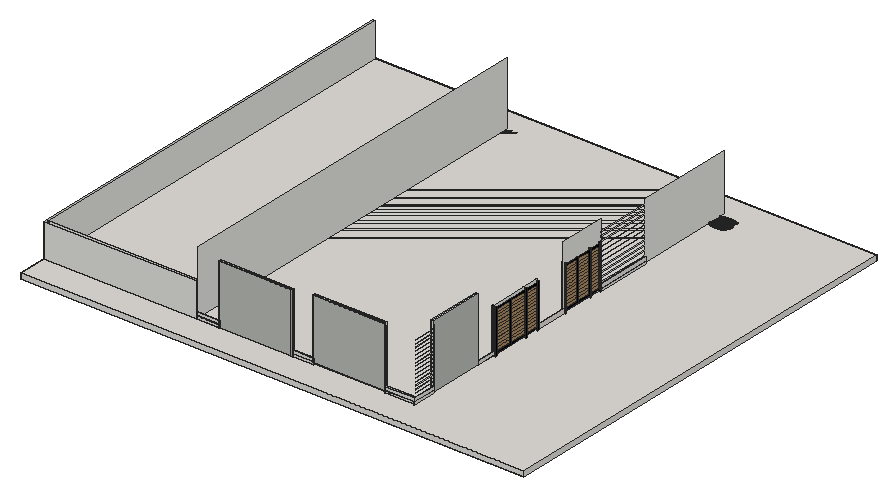
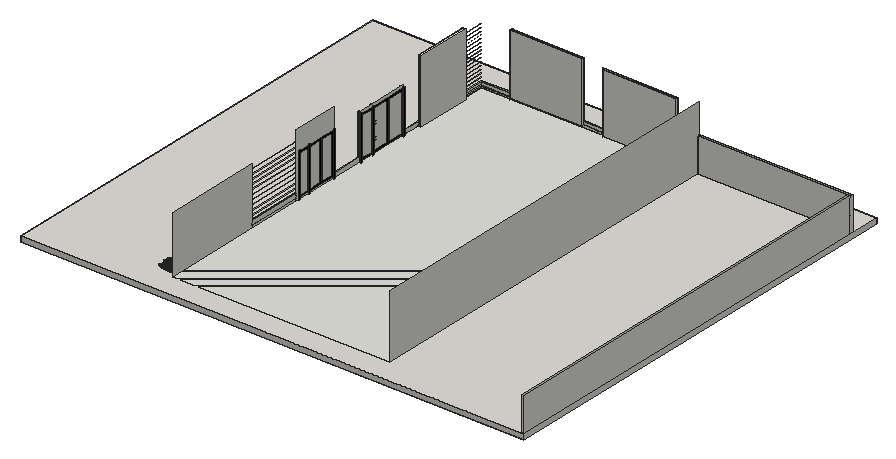
# SketchUp Ruby script. Lengths in inches.
U = 1.inch
M = Sketchup.active_model
def pt(a) = Geom::Point3d.new(a.map { |v| v * U })
def face(e, loops, mat)
  f = e.add_face(loops[0].map { |a| pt(a) })
  loops[1..].each { |l| e.add_face(l.map { |a| pt(a) }).erase! }
  f.material = f.back_material = mat if mat
  f
end
# faces: each face lists its corners as indices into pts; further lists are holes
def faces(e, pts, list, mat = nil) = list.each { |f| face(e, (f[0].is_a?(Array) ? f : [f]).map { |l| l.map { |i| pts[i] } }, mat) }
# xy, xz, yz: faces in a plane at the given z, y or x. An outline is a flat list of corners, or four numbers for a rectangle; further outlines are holes
def ring(l) = l.size == 4 ? [[l[0], l[1]], [l[2], l[1]], [l[2], l[3]], [l[0], l[3]]] : l.each_slice(2).to_a
def flat(e, list, mat, &to3) = list.each { |f| face(e, (f[0].is_a?(Array) ? f : [f]).map { |l| ring(l).map { |u, v| to3.(u, v) } }, mat) }
def xy(e, z, list, mat = nil) = flat(e, list, mat) { |x, y| [x, y, z] }
def xz(e, y, list, mat = nil) = flat(e, list, mat) { |x, z| [x, y, z] }
def yz(e, x, list, mat = nil) = flat(e, list, mat) { |y, z| [x, y, z] }
def lines(e, pts, list) = list.each { |a, b| e.add_line(pt(pts[a]), pt(pts[b])) }
# prism: a flat outline (further loops are holes) pulled along v
def prism(e, loops, v, mat = nil)
  f = face(e, loops, mat); d = Geom::Vector3d.new(v.map { |x| x * U })
  f.pushpull(f.normal.samedirection?(d) ? d.length : -d.length)
end
def box(e, o, s, mat = nil) = prism(e, [[o, [o[0] + s[0], o[1], o[2]], [o[0] + s[0], o[1] + s[1], o[2]], [o[0], o[1] + s[1], o[2]]]], [0, 0, s[2]], mat)
def at(x, y, z, deg = 0) = Geom::Transformation.translation(pt([x, y, z])) * Geom::Transformation.rotation(ORIGIN, Z_AXIS, deg.degrees)
def axes(o, x, y, z) = Geom::Transformation.new([*x, 0, *y, 0, *z, 0, *pt(o).to_a, 1])
def part(name) = M.definitions.add(name)
# library, detail: a bought-in or finely detailed component or shape, given as its bounding box
def library(name, o, s) = part(name).tap { |d| box(d.entities, o, s) }
def detail(e, o, s) = box(e.add_group.entities, o, s)
def put(e, d, t, mat = nil) = e.add_instance(d, t).tap { |i| i.material = mat if mat }
def group(e, t, mat = nil) = e.add_group.tap { |g| g.transformation = t; g.material = mat if mat }.entities
root = M.entities
M.materials.add("CarPaint_Matte_Black").color = [3, 3, 3]
M.materials.add("MaquetteWood_B01_12cm").color = [171, 138, 99]
M.materials.add("Material10").color = [48, 100, 38]
M.materials.add("Material3").color = [68, 110, 58]
M.materials.add("Material4").color = [48, 90, 38]
M.materials.add("Material5").color = [68, 110, 48]
M.materials.add("Material6").color = [48, 90, 48]
M.materials.add("Material7").color = [58, 110, 58]
M.materials.add("Material8").color = [58, 90, 38]
M.materials.add("Material9").color = [68, 100, 58]
M.materials.add("PJ_WallGraphic_V2").color = [185, 188, 181]
M.materials.add("[Terrazzo Tile Accent]").color = [224, 221, 217]
c1 = part("Component\#17")
prism(c1.entities,[[[51.57,0,-2.36],[0,0.39,-2.36],[0.07,5.78,-2.36],[51.65,5.38,-2.36]]],[0,0,82.68])
c2 = part("Component\#14")
prism(c2.entities,[[[1.98,0.39,-2.36],[37.4,0.02,-2.36],[37.4,-0.1,-2.36],[1.98,0.28,-2.36]]],[0,0,82.68],"PJ_WallGraphic_V2")
put(c2.entities,c1,axes([1.98,0,0],[0.68667,0,0],[0,1,0],[0,0,1]))
c3 = part("Gate post")
prism(c3.entities,[[[0,0,0],[3.9375,0,0],[3.9375,0,3.9375],[3.9375,0,98.43],[0,0,98.43]]],[0,7.875,0],"CarPaint_Matte_Black")
c4 = part("Gate post \#2")
box(c4.entities,[0,0,0],[3.9375,7.875,98.43],"CarPaint_Matte_Black")
c5 = part("Gate post \#1")
prism(c5.entities,[[[0,0,0],[3.9375,0,0],[3.9375,0,3.9375],[3.9375,0,98.43],[0,0,98.43]]],[0,7.875,0],"CarPaint_Matte_Black")
c6 = part("Gate leaf frame \#1")
prism(c6.entities,[[[57.09,3.9375,3.9375],[1.97,3.9375,3.9375],[1.97,3.9375,94.49],[57.09,3.9375,94.49]],[[54.13,3.9375,6.89],[54.13,3.9375,91.54],[4.92,3.9375,91.54],[4.92,3.9375,6.89]]],[0,-3.86,0],"CarPaint_Matte_Black")
c7 = part("Gate slat \#1")
box(c7.entities,[0,0,0],[49.21,1.18,5.91],"MaquetteWood_B01_12cm")
c8 = part("Slatted gate panel")
put(c8.entities,c7,at(0,0,25.2))
put(c8.entities,c7,at(0,0,44.09))
put(c8.entities,c7,at(0,0,75.59))
put(c8.entities,c7,at(0,0,69.29))
put(c8.entities,c7,at(0,0,18.9))
put(c8.entities,c7,at(0,0,56.69))
put(c8.entities,c7,at(0,0,50.39))
put(c8.entities,c7,at(0,0,12.6))
put(c8.entities,c7,at(0,0,6.3))
put(c8.entities,c7,at(0,0,37.8))
put(c8.entities,c7,at(0,0,0))
put(c8.entities,c7,at(0,0,31.5))
put(c8.entities,c7,at(0,0,62.99))
c9 = part("Gate leaf frame")
prism(c9.entities,[[[0.98,0,3.9375],[76.39,0,3.9375],[76.39,0,94.49],[0.98,0,94.49]],[[73.43,0,6.89],[3.9375,0,6.89],[3.9375,0,91.54],[73.43,0,91.54]]],[0,3.86,0],"CarPaint_Matte_Black")
c10 = part("Gate slat")
box(c10.entities,[0,0,0],[69.5,1.18,5.91],"MaquetteWood_B01_12cm")
c11 = part("Gate infill panel")
put(c11.entities,c10,at(0,0,56.69))
put(c11.entities,c10,at(0,0,12.6))
put(c11.entities,c10,at(0,0,18.9))
put(c11.entities,c10,at(0,0,37.8))
put(c11.entities,c10,at(0,0,6.3))
put(c11.entities,c10,at(0,0,25.2))
put(c11.entities,c10,at(0,0,75.59))
put(c11.entities,c10,at(0,0,44.09))
put(c11.entities,c10,at(0,0,50.39))
put(c11.entities,c10,at(0,0,0))
put(c11.entities,c10,at(0,0,31.5))
put(c11.entities,c10,at(0,0,62.99))
put(c11.entities,c10,at(0,0,69.29))
c12 = part("Entrance gate assembly")
put(c12.entities,c3,at(0,0,0))
put(c12.entities,c4,at(223.64,0,0))
put(c12.entities,c5,at(160.64,0,0))
g1 = group(c12.entities,at(166.55,2.04,3.9375))
put(g1,c6,at(-1.97,-0.07,-3.9375))
put(g1,c8,at(2.95,1.34,4.33))
g2 = group(c12.entities,at(83.27,2.04,3.9375))
put(g2,c9,at(-0.98,0,-3.9375))
put(g2,c11,at(2.95,1.34,4.33))
g3 = group(c12.entities,at(5.91,2.04,3.9375))
put(g3,c9,axes([76.39,0,-3.9375],[-1,0,0],[0,1,0],[0,0,1]))
put(g3,c11,axes([72.45,1.34,4.33],[-1,0,0],[0,1,0],[0,0,1]))
c13 = part("grass00")
p = [[-0.6875,0.15,0],[-0.56,0.08,5.52],[-0.04,0.03,2.76],[0.48,-0.02,0],[0.35,-0.02,5.52],[-0.1,-0.14,5.52],
  [-0.12,0.65,8.37],[-0.42,0.65,8.37]]
faces(c13.entities,p,[[0,1,2,3],[3,2,4],[1,5,2],[5,4,2],[1,6,5],[4,5,6],[7,6,1]])
c14 = part("Group16\#1")
put(c14.entities,c13,axes([1.44,-0.61,-0.01],[0.05352,0.12609,0],[-0.10704,0.04543,0.07239],[0.06664,-0.02828,0.11628]),"Material6")
put(c14.entities,c13,axes([0.76,-0.15,-0.01],[0.04676,0.24062,0],[-0.23162,0.04501,0.06642],[0.0652,-0.01267,0.23595]),"Material3")
put(c14.entities,c13,axes([0.79,0.01,-0.01],[-0.00606,0.34651,0],[-0.34381,-0.00602,0.0432],[0.04319,0.00076,0.34386]))
put(c14.entities,c13,axes([1,0.23,-0.01],[-0.07192,0.31144,0],[-0.28722,-0.06632,0.1236],[0.12043,0.02781,0.29478]),"Material5")
put(c14.entities,c13,axes([1.66,0.77,-0.01],[-0.13828,0.29651,0],[-0.21551,-0.1005,0.22471],[0.20365,0.09498,0.23779]),"Material10")
put(c14.entities,c13,axes([0.6875,0.52,-0.01],[-0.18126,0.24051,0],[-0.22746,-0.17142,0.09788],[0.07817,0.05891,0.28481]),"Material5")
put(c14.entities,c13,axes([0.68,0.78,-0.01],[-0.215,0.18688,0],[-0.12385,-0.14248,0.21334],[0.13995,0.16101,0.18878]),"Material3")
put(c14.entities,c13,axes([0.56,1,-0.01],[-0.13756,0.07624,0],[-0.06159,-0.11112,0.0927],[0.04494,0.08108,0.12705]),"Material5")
put(c14.entities,c13,axes([0.2,0.64,-0.01],[-0.23729,0.07254,0],[-0.05711,-0.18681,0.153],[0.04473,0.14632,0.19535]),"Material10")
put(c14.entities,c13,axes([0.0625,0.72,-0.01],[-0.28874,0.02525,0],[-0.02179,-0.24916,0.14647],[0.01276,0.14591,0.25012]),"Material3")
put(c14.entities,c13,axes([-0.08,0.62,-0.01],[-0.34089,-0.04187,0],[0.03255,-0.26504,0.216],[-0.02633,0.21439,0.26703]),"Material10")
put(c14.entities,c13,axes([-0.34,0.98,-0.01],[-0.14314,-0.0493,0],[0.04397,-0.12769,0.06843],[-0.02228,0.0647,0.13505]),"Material10")
put(c14.entities,c13,axes([-0.87,1.45,-0.01],[-0.23488,-0.14114,0],[0.13761,-0.22901,0.06087],[-0.03135,0.05217,0.26717]))
put(c14.entities,c13,axes([-0.72,0.77,-0.01],[-0.14208,-0.13251,0],[0.07209,-0.0773,0.16301],[-0.11118,0.11922,0.1057]),"Material10")
put(c14.entities,c13,axes([-0.62,0.43,-0.01],[-0.14845,-0.21203,0],[0.18654,-0.13061,0.12304],[-0.10079,0.07057,0.22772]),"Material3")
put(c14.entities,c13,axes([-0.68,0.29,-0.01],[-0.13639,-0.32136,0],[0.31723,-0.13464,0.05579],[-0.05136,0.0218,0.34462]),"Material4")
put(c14.entities,c13,axes([-0.64,0.125,-0.01],[-0.0458,-0.23569,0],[0.22124,-0.043,0.08276],[-0.08124,0.01579,0.22538]),"Material7")
put(c14.entities,c13,axes([-1.6,-0.03,-0.01],[0.00576,-0.32897,0],[0.27526,0.00482,0.18018],[-0.18015,-0.00315,0.2753]),"Material5")
put(c14.entities,c13,axes([-1.36,-0.31,-0.01],[0.05718,-0.24765,0],[0.18172,0.04196,0.17267],[-0.16825,-0.03885,0.1865]),"Material10")
put(c14.entities,c13,axes([-1.54,-0.72,-0.01],[0.06537,-0.14017,0],[0.13555,0.06321,0.03939],[-0.0357,-0.01665,0.14956]))
put(c14.entities,c13,axes([-1.19,-0.9,-0.01],[0.09597,-0.12735,0],[0.11214,0.08451,0.07557],[-0.06035,-0.04548,0.14042]),"Material9")
put(c14.entities,c13,axes([-0.47,-0.54,-0.01],[0.11588,-0.10072,0],[0.0618,0.0711,0.12124],[-0.07953,-0.0915,0.0942]))
put(c14.entities,c13,axes([-0.47,-0.84,-0.01],[0.11927,-0.0661,0],[0.06603,0.11913,0.00646],[-0.00313,-0.00565,0.13621]),"Material5")
put(c14.entities,c13,axes([-0.38,-1.24,-0.01],[0.28037,-0.08571,0],[0.0618,0.20215,0.20315],[-0.05939,-0.19428,0.21139]),"Material9")
put(c14.entities,c13,axes([-0.06,-0.66,-0.01],[0.22719,-0.01987,0],[0.01247,0.14255,0.17758],[-0.01547,-0.17691,0.1431]),"Material8")
put(c14.entities,c13,axes([0.11,-0.89,-0.01],[0.14882,0.01828,0],[-0.01058,0.08611,0.12229],[0.01491,-0.12138,0.08676]),"Material6")
put(c14.entities,c13,axes([0.25,-0.72,-0.01],[0.20481,0.07053,0],[-0.06206,0.18022,0.10291],[0.03351,-0.0973,0.1906]),"Material6")
put(c14.entities,c13,axes([0.85,-1.42,-0.01],[0.16481,0.09904,0],[-0.09472,0.15762,0.05616],[0.02893,-0.04814,0.18389]),"Material5")
put(c14.entities,c13,axes([1.01,-1.09,-0.01],[0.21858,0.20385,0],[-0.17495,0.1876,0.15339],[0.10462,-0.11218,0.25652]),"Material10")
put(c14.entities,c13,axes([1.01,-0.71,-0.01],[0.08733,0.12473,0],[-0.06445,0.04512,0.13037],[0.1068,-0.07477,0.07867]),"Material6")
c15 = part("Group15\#1")
put(c15.entities,c14,at(0,0,0))
c16 = part("3darcstudiotree_grass00\#1")
put(c16.entities,c15,at(0,0,0))
xy(root,-5.37,[[814.625,599,817.6875,719.91]])
xy(root,-3.47,[[750.91,87.66,750.91,90.47,814.625,90.47,814.625,140.66,816.1875,140.66,816.1875,87.66]])
xy(root,-1.41,[[547.16,87.66,593.34,90.47]])
xy(root,-0.49,[[814.625,423.33,816.875,495.84]])
xy(root,0,[[336.5625,90.47,814.625,939.04]])
xy(root,0.07,[[336.5625,87.66,386.78,90.47]])
xy(root,0.9375,[[814.625,263.05,816.1875,305.04]])
xy(root,3.71,[[750.91,87.66,816.1875,87.66,816.1875,140.66,814.625,140.66,814.625,90.47,750.91,90.47]])
xy(root,3.79,[[814.625,599,817.6875,719.91]])
xy(root,4.59,[[750.91,87.66,750.91,90.47,814.625,90.47,814.625,140.66,816.1875,140.66,816.1875,87.66]])
xy(root,4.76,[[814.625,599,817.6875,719.91]])
xy(root,5.07,[[547.16,87.66,593.34,90.47]])
xy(root,5.21,[[547.16,87.66,593.34,90.47]])
xy(root,6.29,[[336.5625,87.66,386.78,90.47]])
xy(root,6.63,[[336.5625,87.66,386.78,90.47]])
xz(root,87.66,[[0.875,-0.51,0.75,73.42,336.43,74,336.5625,0.07]])
xz(root,87.66,[[750.91,-3.47,816.1875,3.71],[547.16,-1.41,593.34,5.07],[336.5625,0.07,386.78,6.29],[750.91,4.59,816.1875,11.77],[547.16,5.21,593.34,11.69],
  [336.5625,6.63,386.78,12.86]],"[Terrazzo Tile Accent]")
xz(root,90.47,[[336.5625,0,386.78,0.07],[386.78,0,547.16,131.62],[547.16,0,593.34,5.07],[593.34,0,750.91,131.62],[750.91,0,814.625,3.71],
  [336.5625,0.07,386.78,6.29],[750.91,3.71,814.625,4.59],[750.91,4.59,814.625,11.77],[547.16,5.07,593.34,5.21],[547.16,5.21,593.34,11.69],
  [336.5625,6.29,386.78,6.63],[336.5625,6.63,386.78,12.86]])
xz(root,94.42,[[0.875,-0.51,6.22,-0.5,6.1,73.43,0.75,73.42],[6.22,-0.5,336.5625,0.07,336.43,74,6.1,73.43]])
xz(root,140.66,[[814.625,-3.47,816.1875,0],[814.625,0,816.1875,3.71],[814.625,4.59,816.1875,11.77]])
xz(root,263.05,[[814.625,0.9375,816.1875,8.42]])
xz(root,305.04,[[814.625,0.9375,816.1875,8.42]])
xz(root,423.33,[[814.625,-0.49,816.875,8.5]])
xz(root,599,[[814.625,-5.37,817.6875,3.79],[814.625,4.76,817.6875,13.92]])
xz(root,719.91,[[814.625,-5.37,817.6875,3.79],[814.625,4.76,817.6875,13.92]])
yz(root,336.5625,[[90.47,0,939.04,140.0625],[87.66,0.07,90.47,6.29],[87.66,6.63,90.47,12.86]])
yz(root,386.78,[[87.66,0.07,90.47,6.29],[87.66,6.63,90.47,12.86]])
yz(root,547.16,[[87.66,-1.41,90.47,5.07],[87.66,5.21,90.47,11.69]])
yz(root,593.34,[[87.66,-1.41,90.47,5.07],[87.66,5.21,90.47,11.69]])
yz(root,750.91,[[87.66,-3.47,90.47,3.71],[87.66,4.59,90.47,11.77]])
yz(root,814.625,[[87.66,-3.47,87.66,3.71,90.47,3.71,90.47,0,140.66,0,140.66,-3.47],[140.66,0,140.91,0,140.91,131.62,140.66,131.62,140.66,125.4,90.47,125.4,90.47,125.11,140.66,125.11,140.66,117.93,90.47,117.93,90.47,117.55,140.66,117.55,140.66,110.36,90.47,110.36,90.47,110.05,140.66,110.05,140.66,102.86,90.47,102.86,90.47,102.61,140.66,102.61,140.66,95.43,90.47,95.43,90.47,95.17,140.66,95.17,140.66,87.99,90.47,87.99,90.47,87.67,140.66,87.67,140.66,80.49,90.47,80.49,90.47,80.21,140.66,80.21,140.66,73.03,90.47,73.03,90.47,72.77,140.66,72.77,140.66,65.59,90.47,65.59,90.47,65.33,140.66,65.33,140.66,58.15,90.47,58.15,90.47,57.77,140.66,57.77,140.66,50.59,90.47,50.59,90.47,50.15,140.66,50.15,140.66,42.96,90.47,42.96,90.47,42.52,140.66,42.52,140.66,35.34,90.47,35.34,90.47,34.9,140.66,34.9,140.66,27.71,90.47,27.71,90.47,27.27,140.66,27.27,140.66,20.09,90.47,20.09,90.47,19.58,140.66,19.58,140.66,12.4,90.47,12.4,90.47,11.77,140.66,11.77,140.66,4.59,90.47,4.59,90.47,3.71,140.66,3.71],[90.47,0,140.66,3.71],[140.91,0,263.05,131.62],[263.05,0,305.04,0.29],
  [305.04,0,423.33,98.4375],[423.33,0,495.84,8.5],[495.84,0,599,140.0625],[599,0,719.91,3.79],[719.91,0,939.04,0,939.04,125.29,719.91,125.29,719.91,116.13,599,116.13,599,115.17,719.91,115.17,719.91,106.01,599,106.01,599,105.04,719.91,105.04,719.91,95.88,599,95.88,599,94.92,719.91,94.92,719.91,85.76,599,85.76,599,84.79,719.91,84.79,719.91,75.63,599,75.63,599,74.67,719.91,74.67,719.91,65.51,599,65.51,599,64.54,719.91,64.54,719.91,55.38,599,55.38,599,54.42,719.91,54.42,719.91,45.26,599,45.26,599,44.29,719.91,44.29,719.91,35.13,599,35.13,599,34.17,719.91,34.17,719.91,25.01,599,25.01,599,24.04,719.91,24.04,719.91,14.88,599,14.88,599,13.92,719.91,13.92,719.91,4.76,599,4.76,599,3.79,719.91,3.79],
  [263.05,0.29,305.04,0.9375],[263.05,0.9375,305.04,8.42],[90.47,4.59,140.66,11.77],[599,4.76,719.91,13.92]])
yz(root,816.1875,[[87.66,-3.47,140.66,3.71],[263.05,0.9375,305.04,8.42],[87.66,4.59,140.66,11.77]],"[Terrazzo Tile Accent]")
yz(root,816.875,[[423.33,-0.49,495.84,8.5]],"[Terrazzo Tile Accent]")
yz(root,817.6875,[[599,-5.37,719.91,3.79],[599,4.76,719.91,13.92]],"[Terrazzo Tile Accent]")
p = [[0.875,87.66,-0.51],[0.875,94.42,-0.51],[0.75,94.42,73.42],[0.75,87.66,73.42],[0.75,990.97,73.42],[0.875,990.97,-0.51],
  [6.22,94.42,-0.5],[6.22,990.97,-0.5],[6.1,94.42,73.43],[6.1,990.97,73.43],[336.5625,90.47,0.07],[336.5625,87.66,0.07],
  [336.43,87.66,74],[336.43,90.47,74],[336.5625,94.42,0.07],[336.43,94.42,74],[814.625,305.04,0.29],[816.1875,305.04,0.29],
  [814.625,263.05,0.29],[816.1875,263.05,0.29],[6.1,94.42,0]]
faces(root,p,[[0,1,2,3],[1,2,4,5],[6,1,5,7],[8,6,7,9],[10,11,12,13],[14,10,13,15]])
lines(root,p,[[16,17],[18,19],[20,8]])
put(root,c2,axes([376.16,87.76,1.42],[4.494,0,0],[0,1,0],[0,0,1.60205]))
g4 = group(root,at(336.5625,690.47,-12),"[Terrazzo Tile Accent]")
box(g4,[-336.5625,-667.1875,0],[1107.6875,967.6875,12])
put(root,c2,axes([582.64,87.76,7.49],[4.494,0,0],[0,1,0],[0,0,1.60205]))
put(root,c2,axes([814.9,133.37,4],[0,3.46347,0],[-1,0,0],[0,0,1.69406]))
put(root,c12,axes([819.375,305.93,-1.54],[0,0.52,0],[-1,0,0],[0,0,1]))
put(root,c12,axes([819.48,497.55,0],[0,0.4264,0],[-1,0,0],[0,0,1]))
put(root,c16,axes([830.35,906.53,0],[-1.46443,-0.98467,0],[4.53365,-0.42141,-0.02925],[0.15457,-0.01437,1.7044]))
put(root,c16,axes([830.39,898.64,0],[-4.82729,-0.45997,0],[1.31646,-0.86349,-0.04688],[0.11487,-0.07535,1.58936]))
put(root,c16,axes([830.52,899.77,0],[-5.02983,-0.31612,0],[0.92163,-0.91652,-0.02201],[0.03056,-0.03039,1.34565]))
put(root,c16,axes([830.81,923.875,0],[-1.60248,-1.17219,0],[4.18284,-0.35739,-0.03013],[0.15857,-0.01355,1.53631]))
put(root,c16,axes([829.42,893.97,0],[4,0,0],[0,1,0],[0,0,1]))
put(root,c16,axes([829.67,923.15,0],[3.56901,0.48429,0],[-2.2351,1.02948,-0.01651],[-0.0487,0.02243,1.81134]))
put(root,c16,axes([830.52,907.96,0],[-2.03185,0.95693,0],[-3.64296,-0.48344,-0.02935],[-0.13306,-0.01766,1.32321]))
put(root,c16,axes([830.57,901.96,0],[3.55456,-0.14349,0],[0.62802,0.97236,-0.03713],[0.03348,0.05184,1.39317]))
put(root,c16,axes([830.98,921.17,0],[3.6372,-0.13455,0],[0.71258,1.2039,-0.00326],[0.00297,0.00501,1.88794]))
put(root,c16,axes([830.86,895.43,0],[1.65013,1.13441,0],[-3.55007,0.32275,-0.03897],[-0.23777,0.02162,1.53286]))
put(root,c16,axes([833.14,925.85,0],[-5.16631,0.09452,0],[-0.34124,-1.1657,-0.0067],[-0.00219,-0.00748,1.30916]))
put(root,c16,axes([833.88,895.84,0],[2.49255,-0.69469,0],[3.67207,0.82346,-0.03873],[0.17763,0.03983,1.89965]))
put(root,c16,axes([834.4,916.57,0],[-3.93651,0.31096,0],[-1.27927,-1.01217,-0.02199],[-0.03758,-0.02973,1.50537]))
put(root,c16,axes([834.38,913.66,0],[2.99864,-0.87357,0],[3.91675,0.8403,-0.00643],[0.02559,0.00549,1.6911]))
put(root,c16,axes([833.68,906.43,0],[0.74164,0.96677,0],[-4.8523,0.23265,-0.00068],[-0.00352,0.00017,1.62852]))
put(root,c16,axes([835.27,919.3125,0],[1.73951,-1.15891,0],[3.52233,0.33044,-0.02337],[0.15547,0.01459,1.67088]))
put(root,c16,axes([835.66,898.12,0],[-4.02575,0.06277,0],[-0.3115,-1.24857,-0.0193],[-0.00513,-0.02057,1.33558]))
put(root,c16,axes([834.52,897.27,0],[0.21868,1.00492,0],[-3.69218,0.05022,-0.03311],[-0.20682,0.00281,1.44579]))
put(root,c16,axes([835.15,899.51,0],[-2.74984,0.77403,0],[-3.3377,-0.7411,-0.01682],[-0.07048,-0.01565,1.56312]))
put(root,c16,axes([836.16,923.04,0],[-3.8395,0.24007,0],[-0.9565,-0.9561,-0.00789],[-0.01338,-0.01337,1.7222]))
put(root,c16,axes([834.94,902,0],[4.9283,0.10353,0],[-0.353,1.05028,-0.00911],[-0.00564,0.01678,1.94776]))
put(root,c16,axes([836.29,918.45,0],[-3.40628,0.74927,0],[-2.81528,-0.79992,-0.02195],[-0.09915,-0.02817,1.82186]))
put(root,c16,axes([836.8,921.75,0],[2.93374,-0.98597,0],[4.11982,0.76616,-0.01386],[0.04525,0.00841,1.30579]))
put(root,c16,axes([837.42,910.8125,0],[-4.41204,-0.22693,0],[0.9521,-1.15695,-0.02294],[0.02698,-0.03278,1.72347]))
put(root,c16,axes([836.34,907.65,0],[3.69247,-0.55992,0],[2.62164,1.08055,-0.03972],[0.1072,0.04419,1.6444]))
put(root,c16,axes([835.49,924.125,0],[3.49468,0.70982,0],[-2.50295,0.77018,-0.0068],[-0.02397,0.00738,1.38619]))
put(root,c16,axes([835.58,912.08,0],[0.58267,1.0863,0],[-4.76439,0.15972,-0.0098],[-0.05571,0.00187,1.72283]))
put(root,c16,axes([835.72,915.47,0],[4.02178,0.69197,0],[-2.67404,0.97136,-0.05897],[-0.21681,0.07876,1.91169]))
put(root,c16,axes([837.14,904.02,0],[-3.59564,0.7993,0],[-2.95427,-0.83061,-0.01814],[-0.07531,-0.02117,1.73642]))
put(root,c16,axes([837.28,909.42,0],[-3.02071,0.81725,0],[-3.67065,-0.84796,-0.01856],[-0.08057,-0.01861,1.84646]))
put(root,c16,axes([836.86,894.01,0],[4.41696,-0.08184,0],[0.31192,1.05211,-0.02045],[0.01033,0.03484,1.8024]))
put(root,c16,axes([837.38,903.44,0],[1.69404,0.9375,0],[-3.93647,0.44457,-0.01637],[-0.07596,0.00858,1.37485]))
put(root,c16,axes([840.22,900.05,0],[-4.81712,-0.05846,0],[0.24162,-1.24435,-0.01036],[0.00226,-0.01162,1.39846]))
put(root,c16,axes([840.59,918.58,0],[-2.48915,-0.80051,0],[3.17734,-0.61749,-0.04864],[0.28827,-0.05602,1.88819]))
put(root,c16,axes([840.57,905.89,0],[-0.29922,-0.96853,0],[4.43417,-0.08562,-0.04603],[0.2662,-0.00514,1.61216]))
put(root,c16,axes([841.1,920.23,0],[-4.63349,-0.14284,0],[0.49364,-1.00082,-0.03319],[0.02506,-0.0508,1.55524]))
put(root,c16,axes([839.98,912.05,0],[3.90451,-0.09036,0],[0.41259,1.1143,-0.05657],[0.02788,0.07529,1.49576]))
put(root,c16,axes([840.87,913.41,0],[-3.34722,0.62533,0],[-2.16221,-0.72335,-0.01872],[-0.08063,-0.02697,1.62421]))
put(root,c16,axes([841.07,897.39,0],[-3.49291,0.22015,0],[-1.20974,-1.19959,-0.01943],[-0.02054,-0.02037,1.33771]))
put(root,c16,axes([841.68,922.42,0],[-3.43835,-0.52535,0],[2.21532,-0.90619,-0.04274],[0.13952,-0.05707,1.66217]))
put(root,c16,axes([841.82,925.62,0],[-4.50993,0.04391,0],[-0.14231,-0.91361,-0.00954],[-0.0023,-0.01475,1.41434]))
put(root,c16,axes([840.86,924.07,0],[-0.6796,1.05515,0],[-3.94798,-0.15893,-0.03829],[-0.25732,-0.01036,1.70109]))
put(root,c16,axes([842.4,916.64,0],[-0.97949,-1.15886,0],[4.63427,-0.24481,-0.02196],[0.13062,-0.0069,1.79942]))
put(root,c16,axes([840.44,910.19,0],[3.07159,0.54643,0],[-2.5154,0.88372,-0.00585],[-0.0211,0.00741,1.68777]))
put(root,c16,axes([842.01,902,0],[1.11882,-0.9865,0],[3.53965,0.2509,-0.01712],[0.10104,0.00716,1.41054]))
put(root,c16,axes([842.84,909.66,0],[-4.7616,-0.19084,0],[0.68375,-1.06626,-0.05495],[0.05173,-0.08067,1.60563]))
put(root,c16,axes([842.6875,915.17,0],[0.8852,-0.96568,0],[4.22844,0.24225,-0.01662],[0.10834,0.00621,1.81323]))
put(root,c16,axes([841.39,908.03,0],[1.94137,0.91072,0],[-3.56961,0.47558,-0.05193],[-0.33599,0.04476,1.85357]))
put(root,c16,axes([843.08,920.6875,0],[0.57898,-1.02169,0],[3.84832,0.1363,-0.02485],[0.19995,0.00708,1.97391]))
put(root,c16,axes([842.96,895.15,0],[3.44867,-0.28659,0],[1.33447,1.00364,-0.00205],[0.00439,0.0033,1.79239]))
put(root,c16,axes([843.05,898.38,0],[-1.8497,1.19261,0],[-4.37152,-0.42376,-0.03012],[-0.17466,-0.01693,1.82227]))
put(root,c16,axes([843.29,902.53,0],[2.68329,1.05589,0],[-3.47416,0.55179,-0.05376],[-0.29931,0.04754,1.69687]))
put(root,c16,axes([843.37,904.61,0],[4.3739,0.41815,0],[-1.70618,1.11543,-0.01506],[-0.02757,0.01802,1.52965]))
put(root,c16,axes([845.39,899.91,0],[-3.49233,-0.69736,0],[2.36447,-0.74006,-0.04095],[0.19015,-0.05951,1.76156]))
put(root,c16,axes([845.47,901.18,0],[2.09244,-0.94675,0],[3.21681,0.44435,-0.00396],[0.02932,0.00405,1.94458]))
put(root,c16,axes([845.57,903.36,0],[-4.33677,0.62867,0],[-2.01573,-0.86908,-0.01457],[-0.03892,-0.01678,1.33777]))
put(root,c16,axes([845.8,922.98,0],[-1.57293,1.10474,0],[-4.19735,-0.37351,-0.05045],[-0.27865,-0.0248,1.63245]))
put(root,c16,axes([847.37,908.73,0],[-1.17133,-0.98272,0],[4.80109,-0.35766,-0.01047],[0.05653,-0.00421,1.7643]))
